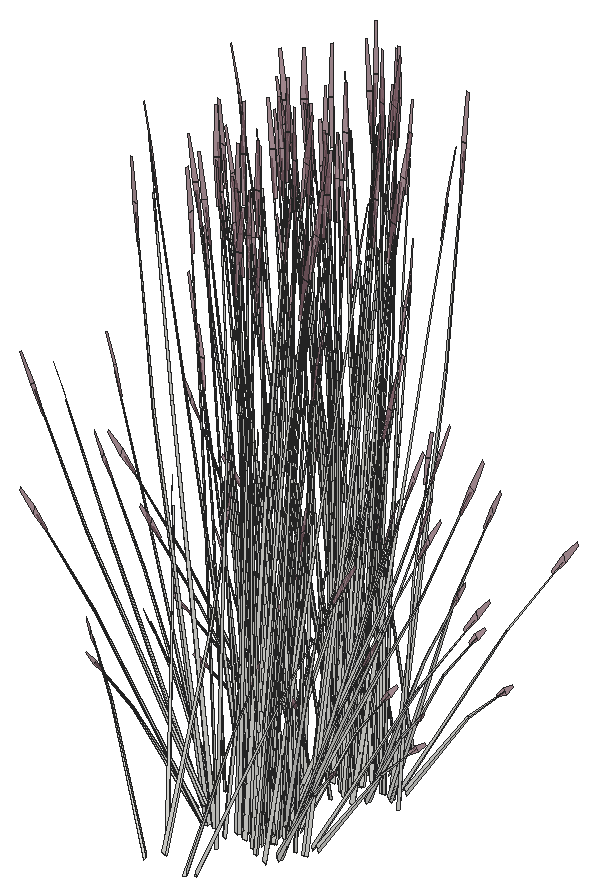
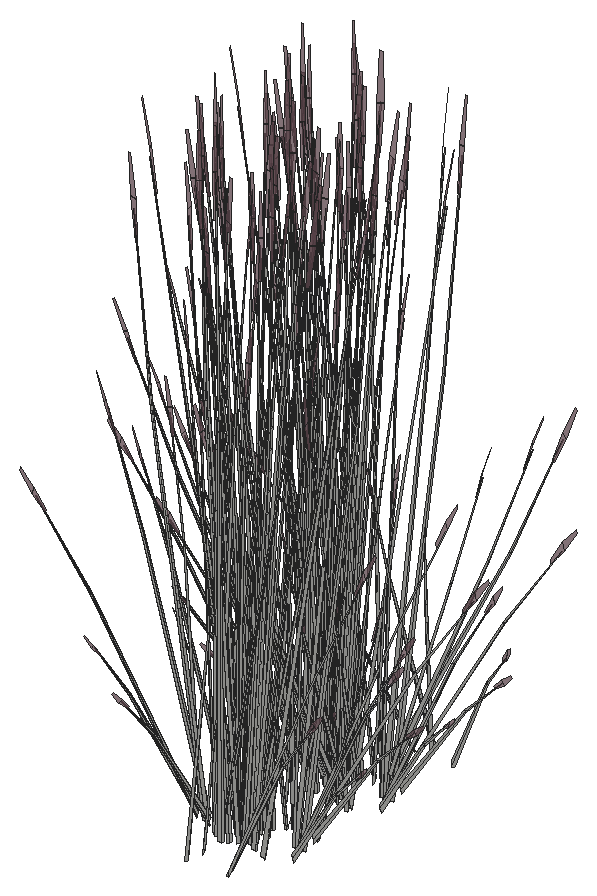
# SketchUp Ruby script. Lengths in inches.
U = 1.inch
M = Sketchup.active_model
def pt(a) = Geom::Point3d.new(a.map { |v| v * U })
def face(e, loops, mat)
  f = e.add_face(loops[0].map { |a| pt(a) })
  loops[1..].each { |l| e.add_face(l.map { |a| pt(a) }).erase! }
  f.material = f.back_material = mat if mat
  f
end
# faces: each face lists its corners as indices into pts; further lists are holes
def faces(e, pts, list, mat = nil) = list.each { |f| face(e, (f[0].is_a?(Array) ? f : [f]).map { |l| l.map { |i| pts[i] } }, mat) }
# xy, xz, yz: faces in a plane at the given z, y or x. An outline is a flat list of corners, or four numbers for a rectangle; further outlines are holes
def ring(l) = l.size == 4 ? [[l[0], l[1]], [l[2], l[1]], [l[2], l[3]], [l[0], l[3]]] : l.each_slice(2).to_a
def flat(e, list, mat, &to3) = list.each { |f| face(e, (f[0].is_a?(Array) ? f : [f]).map { |l| ring(l).map { |u, v| to3.(u, v) } }, mat) }
def xy(e, z, list, mat = nil) = flat(e, list, mat) { |x, y| [x, y, z] }
def xz(e, y, list, mat = nil) = flat(e, list, mat) { |x, z| [x, y, z] }
def yz(e, x, list, mat = nil) = flat(e, list, mat) { |y, z| [x, y, z] }
def lines(e, pts, list) = list.each { |a, b| e.add_line(pt(pts[a]), pt(pts[b])) }
# prism: a flat outline (further loops are holes) pulled along v
def prism(e, loops, v, mat = nil)
  f = face(e, loops, mat); d = Geom::Vector3d.new(v.map { |x| x * U })
  f.pushpull(f.normal.samedirection?(d) ? d.length : -d.length)
end
def box(e, o, s, mat = nil) = prism(e, [[o, [o[0] + s[0], o[1], o[2]], [o[0] + s[0], o[1] + s[1], o[2]], [o[0], o[1] + s[1], o[2]]]], [0, 0, s[2]], mat)
def at(x, y, z, deg = 0) = Geom::Transformation.translation(pt([x, y, z])) * Geom::Transformation.rotation(ORIGIN, Z_AXIS, deg.degrees)
def axes(o, x, y, z) = Geom::Transformation.new([*x, 0, *y, 0, *z, 0, *pt(o).to_a, 1])
def part(name) = M.definitions.add(name)
# library, detail: a bought-in or finely detailed component or shape, given as its bounding box
def library(name, o, s) = part(name).tap { |d| box(d.entities, o, s) }
def detail(e, o, s) = box(e.add_group.entities, o, s)
def put(e, d, t, mat = nil) = e.add_instance(d, t).tap { |i| i.material = mat if mat }
def group(e, t, mat = nil) = e.add_group.tap { |g| g.transformation = t; g.material = mat if mat }.entities
root = M.entities
M.materials.add("LightPink_Translucent").color = [144, 107, 117]
M.materials["LightPink_Translucent"].alpha = 0.75
c1 = part("blade")
p = [[2.15,0.21,22],[0,0.17,0],[0.09,0.45,0],[2.18,0.31,22],[2.29,0.31,22],[0.38,0.45,0],
  [2.48,0.24,33],[2.49,0.24,33],[2.48,0.22,33]]
faces(c1.entities,p,[[0,1,2,3],[4,5,2,3],[6,3,4,7],[8,0,3,6]])
c2 = part("seeds")
p = [[0.3,-0.1,1.38],[-0.01,-0.03,1.59],[-0.01,-0.03,0.03],[0.14,-0.07,-0.07],[0.29,-0.03,3],[0.15,0.01,3.11]]
faces(c2.entities,p,[[0,1,2,3],[1,0,4,5]],"LightPink_Translucent")
c3 = part("blade with seeds")
put(c3.entities,c1,at(0,0,0))
put(c3.entities,c2,axes([2.4,0.25,30.99],[1.5799,-0.05474,1.17369],[-0.12525,1.92788,0.29478],[-0.07173,-0.02425,1.56792]))
put(root,c3,axes([267.875,340.01,124.51],[0.12,0.06519,1.76342],[0.20347,0.60397,-0.26939],[-0.26596,0.12879,0.30037]))
put(root,c3,axes([275.875,346.66,127.3],[0.4673,-0.51481,-0.71045],[0.81887,0.36587,0.08574],[0.27902,-0.18652,1.00501]))
put(root,c3,axes([270.82,345.16,124.7],[-0.55932,-0.6538,0],[0.93577,-0.36461,-0.51607],[0.21313,-0.08304,1.63711]))
put(root,c3,axes([275.85,346.42,127],[-0.22982,-0.59576,-0.51099],[0.87033,-0.10422,-0.3958],[0.24941,-0.16002,0.97773]))
put(root,c3,axes([276.55,346.1875,124.91],[-0.31959,-0.01933,1.43002],[-0.32741,-0.51843,-0.30754],[0.39262,-0.14666,0.61141]))
put(root,c3,axes([273.48,339.19,125.6],[0.01579,-0.21629,1.43002],[0.75442,-0.24159,-0.30754],[0.23289,0.25887,0.61141]))
put(root,c3,axes([276.92,345.24,125.09],[-0.29798,0.33213,1.1486],[-0.25612,-0.44624,0.84392],[0.24611,-0.11182,0.25299]))
put(root,c3,axes([271.58,340.07,124.51],[0.14478,-0.0355,1.76342],[0.8709,0.19542,-0.26939],[0.02547,0.22025,0.30037]))
put(root,c3,axes([268.55,347.49,124.7],[-1.11865,0,0],[0,-0.72922,-0.51607],[0,-0.16609,1.63711]))
put(root,c3,axes([269.57,340.15,125.84],[0.8127,-0.11554,0.06507],[0.18684,0.46549,-0.86304],[-0.05152,0.23564,0.7736]))
put(root,c3,axes([268.74,346.18,124.91],[0.17466,0.18165,1.43002],[-0.40248,0.49377,-0.30754],[-0.41327,-0.11802,0.61141]))
put(root,c3,axes([269.46,346.02,127.3],[-0.89428,-0.01571,-0.71045],[0.06006,-0.66153,0.08574],[-0.37886,-0.06981,1.00501]))
put(root,c3,axes([269.42,347.3,124.65],[-0.83213,0.54855,0.30756],[-0.83263,-0.54278,-0.36492],[-0.02906,-0.15578,1.64885]))
put(root,c3,axes([272.0625,347.55,124.76],[1.00799,0.31623,0.24065],[-0.48511,0.65709,0.50002],[0,-0.15147,1.60543]))
put(root,c3,axes([269.38,340.65,125.6],[0.28231,-0.10293,1.43002],[0.69701,0.31035,-0.30754],[-0.20746,0.26854,0.61141]))
put(root,c3,axes([269.17,346.16,127],[-0.6496,0.4322,-0.51099],[-0.5689,-0.45657,-0.3958],[-0.33005,-0.06576,0.97773]))
put(root,c3,axes([267.7,346.73,125.09],[0.57115,-0.04669,1.1486],[-0.36229,0.41137,0.84392],[-0.28224,-0.06171,0.25299]))
put(root,c3,axes([271.74,347.11,125.04],[-0.97146,0.04028,0.44739],[-0.08785,-0.66859,-0.21531],[0.17391,-0.06776,1.43643]))
put(root,c3,axes([269.23,347.6,124.8],[0,0.65246,0.49651],[-1.00089,0,0],[0,-0.1486,1.57504]))
put(root,c3,axes([276.26,347.74,127],[0.24236,-0.59349,-0.51099],[0.83094,0.20343,-0.3958],[0.33455,-0.05442,0.97773]))
put(root,c3,axes([274.94,345.33,124.7],[0.55932,-0.6538,0],[0.93577,0.36461,-0.51607],[0.21313,0.08304,1.63711]))
put(root,c3,axes([271.7,347.35,124.68],[0.38895,0.72959,0.45755],[-1.11135,0.2537,0.17955],[0.01358,-0.13406,1.58856]))
put(root,c3,axes([271.51,347.93,125.04],[-0.43405,0.58792,0.44739],[-0.90188,-0.28295,-0.21531],[0,-0.13553,1.43643]))
put(root,c3,axes([273.1,347.41,124.53],[0,-0.75495,0],[1.11865,0,0],[0,0,1.79456]))
put(root,c3,axes([274.46,345.67,124.8],[-0.83726,-0.32623,0.49651],[0.50045,-0.58498,0],[0.19069,0.0743,1.57504]))
put(root,c3,axes([276.1,347.96,127.3],[0.78611,-0.28816,-0.71045],[0.4381,0.59317,0.08574],[0.37982,-0.06738,1.00501]))
put(root,c3,axes([272.57,346.9375,124.68],[-0.74176,0.59212,0.45755],[-0.88124,-0.52269,0.17955],[0.17882,-0.05909,1.58856]))
put(root,c3,axes([273.38,348,124.62],[-0.83213,-0.56158,-0.06131],[0.83263,-0.56193,0],[-0.02906,-0.01961,1.75571]))
put(root,c3,axes([271.29,345.96,124.8],[-0.25843,0.64844,0.17642],[-0.9457,-0.1835,0.35086],[0.16336,-0.00316,1.60407]))
put(root,c3,axes([273.26,346.68,124.94],[0.17258,-0.58229,0.1448],[0.84319,0.10108,-0.41347],[0.15345,0.05979,1.26744]))
put(root,c3,axes([271.8,348.07,124.68],[1.13071,0.13747,0.45755],[-0.23011,0.77639,0.17955],[-0.16524,-0.07497,1.58856]))
put(root,c3,axes([272.9,346.84,125.04],[-0.53742,-0.54764,0.44739],[0.81403,-0.38564,-0.21531],[0.17391,0.06776,1.43643]))
put(root,c3,axes([271.19,349.31,124.8],[0.96132,-0.17317,0.17642],[0.23737,0.64447,0.35086],[-0.08574,-0.0939,1.60407]))
put(root,c3,axes([273.86,347.58,124.53],[1.00089,0,0],[0,0.67548,0],[0,0,1.78407]))
put(root,c3,axes([274.15,346,124.8],[-0.96132,0.17317,0.17642],[-0.23737,-0.64447,0.35086],[0.08574,0.0939,1.60407]))
put(root,c3,axes([273.54,347.24,124.7],[-1.13071,-0.13747,0.49198],[0.23011,-0.77639,0.19306],[0.16524,0.07497,1.70813]))
put(root,c3,axes([272.64,349.15,124.53],[-0.29189,-0.56252,0],[0.83351,-0.19699,0],[0,0,1.54371]))
put(root,c3,axes([272.08,348.62,124.94],[-0.17258,0.58229,0.1448],[-0.84319,-0.10108,-0.41347],[-0.15345,-0.05979,1.26744]))
put(root,c3,axes([274.05,349.34,124.8],[0.25843,-0.64844,0.17642],[0.9457,0.1835,0.35086],[-0.16336,0.00316,1.60407]))
put(root,c3,axes([273.84,347.87,124.54],[0.62448,0.42144,0],[-0.62448,0.42144,0],[0,0,1.69266]))
put(root,c3,axes([275.53,347.6875,124.8],[-0.70288,-0.47526,0.17642],[0.70832,-0.46097,0.35086],[-0.07763,0.09706,1.60407]))
put(root,c3,axes([278.34,348.12,125.09],[-0.55274,0.10771,1.1486],[0.26018,-0.44517,0.84392],[0.29323,0.03046,0.25299]))
put(root,c3,axes([272.43,349.41,124.52],[-0.90188,-0.29293,0],[0.43405,-0.60866,0],[0,0,1.62707]))
put(root,c3,axes([270.88,349.64,124.8],[0.83726,0.32623,0.49651],[-0.50045,0.58498,0],[-0.19069,-0.0743,1.57504]))
put(root,c3,axes([273.83,347.38,125.04],[0.43405,-0.58792,0.44739],[0.90188,0.28295,-0.21531],[0,0.13553,1.43643]))
put(root,c3,axes([273.67,347.71,124.62],[0,0.75458,-0.05637],[-1.11865,0,0],[0,0.02371,1.79368]))
put(root,c3,axes([268.54,347.44,127],[-0.24236,0.59349,-0.51099],[-0.83094,-0.20343,-0.3958],[-0.33455,0.05442,0.97773]))
put(root,c3,axes([270.4,349.98,124.7],[-0.55932,0.6538,0],[-0.93577,-0.36461,-0.51607],[-0.21313,-0.08304,1.63711]))
put(root,c3,axes([276.11,347.71,124.8],[0,-0.65246,0.49651],[1.00089,0,0],[0,0.1486,1.57504]))
put(root,c3,axes([273.6,348.19,125.04],[0.97146,-0.04028,0.44739],[0.08785,0.66859,-0.21531],[-0.17391,0.06776,1.43643]))
put(root,c3,axes([274.21,347.51,124.94],[0.83351,-0.19028,0.1448],[0.29189,0.54335,-0.41347],[0,0.11958,1.26744]))
put(root,c3,axes([277.31,348.84,124.91],[-0.21545,-0.16047,1.43002],[0.28033,-0.53085,-0.30754],[0.43591,0.07191,0.61141]))
put(root,c3,axes([273.45,349.42,124.53],[0.90188,0.29293,0],[-0.43405,0.60866,0],[0,0,1.74954]))
put(root,c3,axes([274.1,355.17,125.24],[-0.25429,0.13207,1.43002],[-0.76157,-0.23115,-0.30754],[0.14117,-0.28747,0.61141]))
put(root,c3,axes([273.62,348.48,124.94],[0.66093,0.39201,0.1448],[-0.5513,0.44227,-0.41347],[-0.15345,0.05979,1.26744]))
put(root,c3,axes([270.16,354.92,125.24],[-0.05417,0.21344,1.43002],[-0.79196,0.17867,-0.30754],[-0.18512,-0.27588,0.61141]))
put(root,c3,axes([275.33,349.16,127.3],[0.89428,0.01571,-0.71045],[-0.06006,0.66153,0.08574],[0.37886,0.06981,1.00501]))
put(root,c3,axes([274.32,349.69,124.8],[0.83726,-0.32623,0.49651],[0.50045,0.58498,0],[-0.19069,0.0743,1.57504]))
put(root,c3,axes([273.13,349.17,124.61],[0.38895,0.74956,-0.06012],[-1.11135,0.26265,0],[0.01358,0.02618,1.72173]))
put(root,c3,axes([267.54,348.83,124.91],[0.3109,0.05356,1.43002],[0.20038,0.54709,-0.30754],[-0.42231,0.10241,0.61141]))
put(root,c3,axes([276.79,347.82,124.7],[1.11865,0,0],[0,0.72922,-0.51607],[0,0.16609,1.63711]))
put(root,c3,axes([273.16,354.12,125.41],[0.11476,0.38047,1.1486],[-0.63664,-0.21072,0.84392],[0.06851,-0.19481,0.25299]))
put(root,c3,axes([266.89,349.98,125.09],[0.37283,-0.29571,1.1486],[0.14711,0.46813,0.84392],[-0.26943,0.08382,0.25299]))
put(root,c3,axes([269.89,354.58,125.41],[0.46666,0.22709,1.1486],[-0.67962,0.13651,0.84392],[-0.14541,-0.17452,0.25299]))
put(root,c3,axes([273.84,349.73,124.65],[1.11998,0.21207,0.30756],[-0.2802,0.75803,-0.36492],[-0.18537,0.09487,1.64885]))
put(root,c3,axes([275.27,349.67,125.09],[-0.5037,-0.18761,1.1486],[0.6504,-0.19062,0.84392],[0.17543,0.16147,0.25299]))
put(root,c3,axes([268.94,348.76,127],[0.22982,0.59576,-0.51099],[-0.87033,0.10422,-0.3958],[-0.24941,0.16002,0.97773]))
put(root,c3,axes([274.52,350.14,124.7],[0.55932,0.6538,0],[-0.93577,0.36461,-0.51607],[-0.21313,0.08304,1.63711]))
put(root,c3,axes([274.04,347.55,125.17],[-0.02444,-0.61432,1.41272],[1.10603,0.15924,0.59816],[-0.26159,0.33615,1.3335]))
put(root,c3,axes([274.13,349.92,127],[0.88277,-0.1551,-0.51099],[0.15442,0.58737,-0.3958],[0.23711,0.16832,0.97773]))
put(root,c3,axes([270.82,355.7,125.02],[-0.55932,-0.6538,0],[0.93577,-0.36461,-0.51607],[0.21313,-0.08304,1.63711]))
put(root,c3,axes([275.35,350.52,124.99],[-0.57368,-0.02046,1.0506],[0.37886,-0.43461,0.58006],[0.22663,0.15441,0.8241]))
put(root,c3,axes([272.05,354.91,124.77],[-0.61821,0.37431,-0.03893],[-0.56645,-0.40995,-0.17649],[-0.03988,-0.11616,0.58215]))
put(root,c3,axes([273.48,349.47,124.91],[0.01579,-0.21629,1.43002],[0.75442,-0.24159,-0.30754],[0.23289,0.25887,0.61141]))
put(root,c3,axes([276.55,356.72,125.24],[-0.31959,-0.01933,1.43002],[-0.32741,-0.51843,-0.30754],[0.39262,-0.14666,0.61141]))
put(root,c3,axes([270.05,351.27,125.09],[-0.02315,-0.38796,1.1486],[0.57853,0.27671,0.84392],[-0.11378,0.18492,0.25299]))
put(root,c3,axes([276.92,355.77,125.41],[-0.29798,0.33213,1.1486],[-0.25612,-0.44624,0.84392],[0.24611,-0.11182,0.25299]))
put(root,c3,axes([269.57,350.43,125.15],[0.8127,-0.11554,0.06507],[0.18684,0.46549,-0.86304],[-0.05152,0.23564,0.7736]))
put(root,c3,axes([272.17,350.2,127],[0.87941,0.16356,-0.51099],[-0.30143,0.56078,-0.3958],[0.08064,0.22578,0.97773]))
put(root,c3,axes([268.98,355.59,124.77],[-0.25807,0.53277,-0.03893],[-0.79428,-0.16389,-0.17649],[-0.1206,-0.08714,0.58215]))
put(root,c3,axes([268.55,358.02,125.02],[-1.11865,0,0],[0,-0.72922,-0.51607],[0,-0.16609,1.63711]))
put(root,c3,axes([268.74,356.72,125.24],[0.17466,0.18165,1.43002],[-0.40248,0.49377,-0.30754],[-0.41327,-0.11802,0.61141]))
put(root,c3,axes([270.07,349.57,127.66],[-0.02328,0.60353,-0.7886],[-0.98022,-0.04053,0.09517],[-0.10344,0.25568,1.11556]))
put(root,c3,axes([271.85,350.09,127.3],[0.42698,0.53052,-0.71045],[-0.87893,0.29566,0.08574],[0.09984,0.25633,1.00501]))
put(root,c3,axes([269.42,357.83,124.98],[-0.83213,0.54855,0.30756],[-0.83263,-0.54278,-0.36492],[-0.02906,-0.15578,1.64885]))
put(root,c3,axes([269.38,350.92,124.91],[0.28231,-0.10293,1.43002],[0.69701,0.31035,-0.30754],[-0.20746,0.26854,0.61141]))
put(root,c3,axes([272.0625,358.09,125.08],[1.00799,0.31623,0.24065],[-0.48511,0.65709,0.50002],[0,-0.15147,1.60543]))
put(root,c3,axes([271.67,358.97,125.08],[0.23711,-0.77313,-0.23429],[1.12425,0.13477,0.51271],[-0.19645,-0.10677,1.5644]))
put(root,c3,axes([267.7,357.27,125.41],[0.57115,-0.04669,1.1486],[-0.36229,0.41137,0.84392],[-0.28224,-0.06171,0.25299]))
put(root,c3,axes([271.74,357.65,125.36],[-0.97146,0.04028,0.44739],[-0.08785,-0.66859,-0.21531],[0.17391,-0.06776,1.43643]))
put(root,c3,axes([269.23,358.13,125.125],[0,0.65246,0.49651],[-1.00089,0,0],[0,-0.1486,1.57504]))
put(root,c3,axes([274.94,355.86,125.02],[0.55932,-0.6538,0],[0.93577,0.36461,-0.51607],[0.21313,0.08304,1.63711]))
put(root,c3,axes([271.7,357.89,125.01],[0.38895,0.72959,0.45755],[-1.11135,0.2537,0.17955],[0.01358,-0.13406,1.58856]))
put(root,c3,axes([277.14,358.45,124.63],[-0.57619,0.0783,1.41583],[-0.09171,-0.62326,0.08104],[0.40356,-0.09434,0.80566]))
put(root,c3,axes([278.19,357.89,124.91],[-0.55463,-0.41721,-0.06488],[0.60744,-0.38228,-0.29416],[0.17212,-0.02691,0.97024]))
put(root,c3,axes([271.51,358.46,125.36],[-0.43405,0.58792,0.44739],[-0.90188,-0.28295,-0.21531],[0,-0.13553,1.43643]))
put(root,c3,axes([273.1,357.95,124.85],[0,-0.75495,0],[1.11865,0,0],[0,0,1.79456]))
put(root,c3,axes([274.46,356.2,125.125],[-0.83726,-0.32623,0.49651],[0.50045,-0.58498,0],[0.19069,0.0743,1.57504]))
put(root,c3,axes([272.57,357.47,125.01],[-0.74176,0.59212,0.45755],[-0.88124,-0.52269,0.17955],[0.17882,-0.05909,1.58856]))
put(root,c3,axes([273.38,358.53,124.94],[-0.83213,-0.56158,-0.06131],[0.83263,-0.56193,0],[-0.02906,-0.01961,1.75571]))
put(root,c3,axes([271.29,356.5,125.12],[-0.25843,0.64844,0.17642],[-0.9457,-0.1835,0.35086],[0.16336,-0.00316,1.60407]))
put(root,c3,axes([273.26,357.22,125.26],[0.17258,-0.58229,0.1448],[0.84319,0.10108,-0.41347],[0.15345,0.05979,1.26744]))
put(root,c3,axes([271.8,358.6,125.01],[1.13071,0.13747,0.45755],[-0.23011,0.77639,0.17955],[-0.16524,-0.07497,1.58856]))
put(root,c3,axes([272.9,357.37,125.36],[-0.53742,-0.54764,0.44739],[0.81403,-0.38564,-0.21531],[0.17391,0.06776,1.43643]))
put(root,c3,axes([271.19,359.84,125.12],[0.96132,-0.17317,0.17642],[0.23737,0.64447,0.35086],[-0.08574,-0.0939,1.60407]))
put(root,c3,axes([273.86,358.12,124.85],[1.00089,0,0],[0,0.67548,0],[0,0,1.78407]))
put(root,c3,axes([274.15,356.53,125.12],[-0.96132,0.17317,0.17642],[-0.23737,-0.64447,0.35086],[0.08574,0.0939,1.60407]))
put(root,c3,axes([273.54,357.77,125.03],[-1.13071,-0.13747,0.49198],[0.23011,-0.77639,0.19306],[0.16524,0.07497,1.70813]))
put(root,c3,axes([272.64,359.69,124.85],[-0.29189,-0.56252,0],[0.83351,-0.19699,0],[0,0,1.54371]))
put(root,c3,axes([272.08,359.16,125.26],[-0.17258,0.58229,0.1448],[-0.84319,-0.10108,-0.41347],[-0.15345,-0.05979,1.26744]))
put(root,c3,axes([274.05,359.88,125.12],[0.25843,-0.64844,0.17642],[0.9457,0.1835,0.35086],[-0.16336,0.00316,1.60407]))
put(root,c3,axes([273.84,358.41,124.86],[0.62448,0.42144,0],[-0.62448,0.42144,0],[0,0,1.69266]))
put(root,c3,axes([275.53,358.22,125.12],[-0.70288,-0.47526,0.17642],[0.70832,-0.46097,0.35086],[-0.07763,0.09706,1.60407]))
put(root,c3,axes([278.34,358.66,125.41],[-0.55274,0.10771,1.1486],[0.26018,-0.44517,0.84392],[0.29323,0.03046,0.25299]))
put(root,c3,axes([272.43,359.94,124.84],[-0.90188,-0.29293,0],[0.43405,-0.60866,0],[0,0,1.62707]))
put(root,c3,axes([270.88,360.17,125.125],[0.83726,0.32623,0.49651],[-0.50045,0.58498,0],[-0.19069,-0.0743,1.57504]))
put(root,c3,axes([273.83,357.91,125.36],[0.43405,-0.58792,0.44739],[0.90188,0.28295,-0.21531],[0,0.13553,1.43643]))
put(root,c3,axes([273.67,358.25,124.9375],[0,0.75458,-0.05637],[-1.11865,0,0],[0,0.02371,1.79368]))
put(root,c3,axes([270.4,360.51,125.02],[-0.55932,0.6538,0],[-0.93577,-0.36461,-0.51607],[-0.21313,-0.08304,1.63711]))
put(root,c3,axes([274.1,364.99,125.27],[-0.25429,0.13207,1.43002],[-0.76157,-0.23115,-0.30754],[0.14117,-0.28747,0.61141]))
put(root,c3,axes([276.11,358.24,125.125],[0,-0.65246,0.49651],[1.00089,0,0],[0,0.1486,1.57504]))
put(root,c3,axes([273.6,358.73,125.36],[0.97146,-0.04028,0.44739],[0.08785,0.66859,-0.21531],[-0.17391,0.06776,1.43643]))
put(root,c3,axes([274.21,358.05,125.26],[0.83351,-0.19028,0.1448],[0.29189,0.54335,-0.41347],[0,0.11958,1.26744]))
put(root,c3,axes([270.16,364.74,125.27],[-0.05417,0.21344,1.43002],[-0.79196,0.17867,-0.30754],[-0.18512,-0.27588,0.61141]))
put(root,c3,axes([277.31,359.37,125.24],[-0.21545,-0.16047,1.43002],[0.28033,-0.53085,-0.30754],[0.43591,0.07191,0.61141]))
put(root,c3,axes([273.45,359.96,124.85],[0.90188,0.29293,0],[-0.43405,0.60866,0],[0,0,1.74954]))
put(root,c3,axes([273.8125,360.6,124.84],[-0.55235,-0.65609,-0.05142],[0.93577,-0.36461,0.51607],[-0.23059,0.06247,1.6363]))
put(root,c3,axes([273.62,359.02,125.26],[0.66093,0.39201,0.1448],[-0.5513,0.44227,-0.41347],[-0.15345,0.05979,1.26744]))
put(root,c3,axes([273.16,363.94,125.44],[0.11476,0.38047,1.1486],[-0.63664,-0.21072,0.84392],[0.06851,-0.19481,0.25299]))
put(root,c3,axes([274.32,360.23,125.125],[0.83726,-0.32623,0.49651],[0.50045,0.58498,0],[-0.19069,0.0743,1.57504]))
put(root,c3,axes([273.13,359.71,124.9375],[0.38895,0.74956,-0.06012],[-1.11135,0.26265,0],[0.01358,0.02618,1.72173]))
put(root,c3,axes([267.54,359.37,125.24],[0.3109,0.05356,1.43002],[0.20038,0.54709,-0.30754],[-0.42231,0.10241,0.61141]))
put(root,c3,axes([276.79,358.35,125.02],[1.11865,0,0],[0,0.72922,-0.51607],[0,0.16609,1.63711]))
put(root,c3,axes([276.34,358.73,124.84],[-1.1181,-0.00522,-0.04976],[0,-0.72922,0.49943],[-0.03514,0.166,1.58352]))
put(root,c3,axes([269.89,364.4,125.44],[0.46666,0.22709,1.1486],[-0.67962,0.13651,0.84392],[-0.14541,-0.17452,0.25299]))
put(root,c3,axes([266.89,360.51,125.41],[0.37283,-0.29571,1.1486],[0.14711,0.46813,0.84392],[-0.26943,0.08382,0.25299]))
put(root,c3,axes([273.84,360.27,124.98],[1.11998,0.21207,0.30756],[-0.2802,0.75803,-0.36492],[-0.18537,0.09487,1.64885]))
put(root,c3,axes([275.27,360.2,125.41],[-0.5037,-0.18761,1.1486],[0.6504,-0.19062,0.84392],[0.17543,0.16147,0.25299]))
